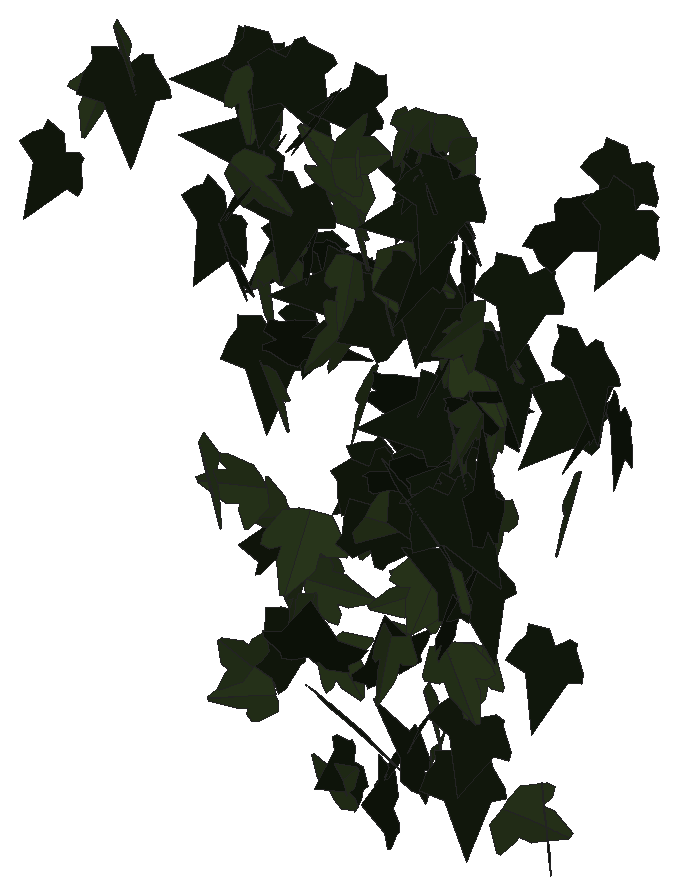
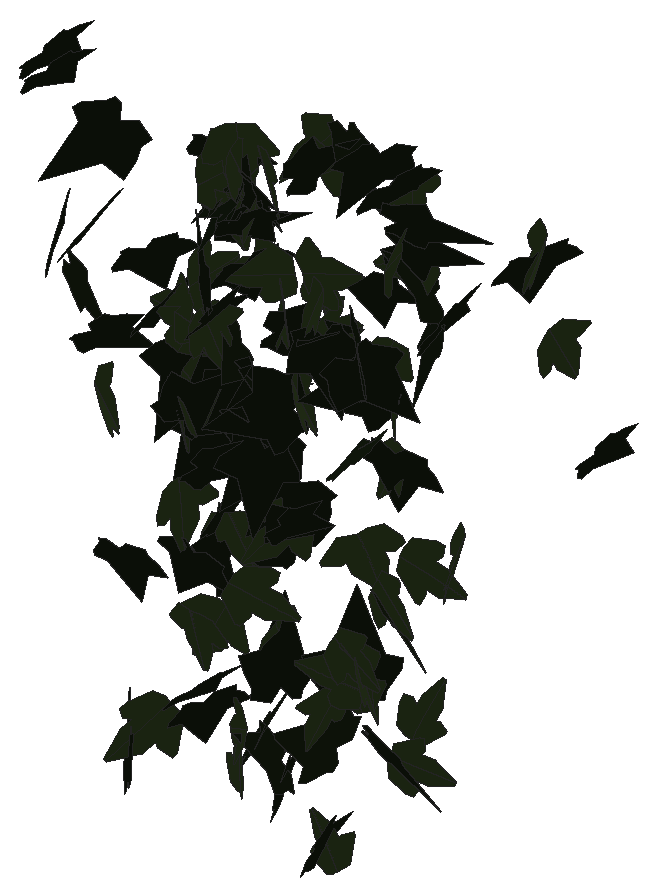
# SketchUp Ruby script. Lengths in inches.
U = 1.inch
M = Sketchup.active_model
def pt(a) = Geom::Point3d.new(a.map { |v| v * U })
def face(e, loops, mat)
  f = e.add_face(loops[0].map { |a| pt(a) })
  loops[1..].each { |l| e.add_face(l.map { |a| pt(a) }).erase! }
  f.material = f.back_material = mat if mat
  f
end
# faces: each face lists its corners as indices into pts; further lists are holes
def faces(e, pts, list, mat = nil) = list.each { |f| face(e, (f[0].is_a?(Array) ? f : [f]).map { |l| l.map { |i| pts[i] } }, mat) }
# xy, xz, yz: faces in a plane at the given z, y or x. An outline is a flat list of corners, or four numbers for a rectangle; further outlines are holes
def ring(l) = l.size == 4 ? [[l[0], l[1]], [l[2], l[1]], [l[2], l[3]], [l[0], l[3]]] : l.each_slice(2).to_a
def flat(e, list, mat, &to3) = list.each { |f| face(e, (f[0].is_a?(Array) ? f : [f]).map { |l| ring(l).map { |u, v| to3.(u, v) } }, mat) }
def xy(e, z, list, mat = nil) = flat(e, list, mat) { |x, y| [x, y, z] }
def xz(e, y, list, mat = nil) = flat(e, list, mat) { |x, z| [x, y, z] }
def yz(e, x, list, mat = nil) = flat(e, list, mat) { |y, z| [x, y, z] }
def lines(e, pts, list) = list.each { |a, b| e.add_line(pt(pts[a]), pt(pts[b])) }
# prism: a flat outline (further loops are holes) pulled along v
def prism(e, loops, v, mat = nil)
  f = face(e, loops, mat); d = Geom::Vector3d.new(v.map { |x| x * U })
  f.pushpull(f.normal.samedirection?(d) ? d.length : -d.length)
end
def box(e, o, s, mat = nil) = prism(e, [[o, [o[0] + s[0], o[1], o[2]], [o[0] + s[0], o[1] + s[1], o[2]], [o[0], o[1] + s[1], o[2]]]], [0, 0, s[2]], mat)
def at(x, y, z, deg = 0) = Geom::Transformation.translation(pt([x, y, z])) * Geom::Transformation.rotation(ORIGIN, Z_AXIS, deg.degrees)
def axes(o, x, y, z) = Geom::Transformation.new([*x, 0, *y, 0, *z, 0, *pt(o).to_a, 1])
def part(name) = M.definitions.add(name)
# library, detail: a bought-in or finely detailed component or shape, given as its bounding box
def library(name, o, s) = part(name).tap { |d| box(d.entities, o, s) }
def detail(e, o, s) = box(e.add_group.entities, o, s)
def put(e, d, t, mat = nil) = e.add_instance(d, t).tap { |i| i.material = mat if mat }
def group(e, t, mat = nil) = e.add_group.tap { |g| g.transformation = t; g.material = mat if mat }.entities
root = M.entities
M.materials.add("efeu1").color = [18, 25, 13]
M.materials.add("efeu2").color = [43, 57, 29]
c1 = part("ivyleaf_10")
p = [[0,0.5,-0.03],[-0.0625,2.02,-0.43],[-0.19,2.01,-0.46],[-0.54,1.05,-0.29],[-0.52,0.625,-0.18],[-0.83,0.76,-0.28],
  [-1.16,0.64,-0.33],[-1.15,0.33,-0.24],[-0.77,-0.39,0.02],[-0.3,-0.51,0.16],[0.04,-0.48,0.23],[-0.02,2.01,-0.4375],
  [-0.06,2.01,-0.43],[0.04,-0.49,0.23],[0.67,-0.49,0.14],[1.38,0.36,-0.2],[1.375,0.51,-0.24],[0.81,0.65,-0.19],
  [0.62,0.59,-0.15],[0.6,1.09,-0.28],[0.5,1.23,-0.31]]
faces(c1.entities,p,[[0,1,2,3,4,5,6,7,8,9,10],[11,12,0,13,14,15,16,17,18,19,20]],"efeu2")
c2 = part("ivyleaf_9")
p = [[1.54,2.16,1.25],[1.36,2.04,1.19],[-0.21,0.99,0.68],[-0.71,1.11,0.82],[-0.85,0.86,0.67],[-0.8,0.17,0.21],
  [-0.9,-0.01,0.1],[-0.67,-0.16,-0.02],[-0.08,-0.08,-0.05],[-0.03,-0.6,-0.4],[0.65,-0.88,-0.66],[0.83,-0.6,-0.49],
  [1.29,-0.42,-0.43],[1.8125,-0.07,-0.26],[1.21,0.44,0.15]]
faces(c2.entities,p,[[0,1,2,3,4,5,6,7,8,9,10,11,12,13,14]],"efeu1")
put(root,c1,axes([506.54,130.52,199.08],[-0.00627,-0.15637,0.93433],[0.25618,-0.86774,-0.15548],[0.95095,0.23273,0.04805]))
put(root,c1,axes([503.25,130.37,187.29],[-0.25922,-0.47722,-0.5607],[-0.25918,-0.48278,0.55554],[-0.73314,0.3394,0.00185]))
put(root,c1,axes([505.48,130.12,192.53],[0.69257,0.65461,-0.29515],[-0.19639,-0.21903,-0.95275],[-0.74512,0.66618,-0.02322]))
put(root,c2,axes([502.125,130.74,201.16],[-0.14431,-0.75939,0.55347],[-0.07524,-0.52794,-0.80165],[0.99866,-0.14951,0.01958]))
put(root,c1,axes([506.75,130.1,204.41],[0.54661,0.1085,0.66627],[-0.67489,-0.14122,0.5383],[0.19227,-0.80414,-0.00464]))
put(root,c2,axes([512.3,129.8,195.1],[-0.12147,-0.53915,0.79492],[0.15053,0.78066,0.55249],[-0.94864,0.19291,-0.01411]))
put(root,c1,axes([501.97,130.09,193.54],[-0.52665,0.83056,-0.10382],[0.04851,-0.08939,-1.00163],[-0.90216,-0.48966,0.00675]))
put(root,c2,axes([510.1,130.49,203.04],[-0.89494,0.25895,-0.37431],[0.36721,-0.1185,-0.90282],[-0.30734,-0.89562,0.01123]))
put(root,c1,axes([506.82,130.43,201.11],[0.79198,-0.33689,0.12485],[0.11865,-0.04842,-0.83928],[0.36757,0.7415,0.00191]))
put(root,c2,axes([505.98,130.14,205.92],[-0.44026,0.68291,-0.04296],[0.01968,-0.03722,-0.82713],[-0.73863,-0.40804,0.00356]))
put(root,c2,axes([508.62,130.63,194.77],[0.64339,-0.64937,0.36279],[0.24199,-0.27085,-0.91396],[0.70338,0.68717,-0.01741]))
put(root,c2,axes([516.2,130.92,199.53],[0.14807,-0.04382,-0.8756],[0.76524,-0.42684,0.15077],[-0.42778,-0.77872,-0.03337]))
put(root,c2,axes([505.23,130.65,188.13],[0.95979,0.11256,0.3282],[-0.33969,-0.02795,0.93156],[0.12468,-0.94265,0.01157]))
put(root,c1,axes([503.05,130.43,203.03],[-0.43402,0.06889,-0.75913],[0.77065,-0.15446,-0.42374],[-0.1819,-0.8188,0.01606]))
put(root,c2,axes([498.62,130.75,204.66],[-0.16588,-0.89543,-0.19328],[0.03476,0.18304,-0.94485],[0.98706,-0.15692,0.00079]))
put(root,c2,axes([502.73,130.12,200.56],[0.58447,-0.12641,-0.61836],[-0.60118,0.21677,-0.57485],[0.26375,0.77421,0.05999]))
put(root,c1,axes([507.24,129.79,205.2],[-0.0469,0.24958,0.915],[-0.14978,0.86881,-0.26344],[-0.97626,-0.14529,-0.00354]))
put(root,c1,axes([503.45,130.76,186.16],[-0.14934,-0.06886,0.76036],[-0.64128,-0.42726,-0.15865],[0.46665,-0.60918,0.02532]))
put(root,c2,axes([510.42,130.52,195],[-0.10303,-0.62569,-0.77186],[0.22837,0.74031,-0.6306],[0.96701,-0.2415,0.06668]))
put(root,c1,axes([503.16,130.58,192.85],[0.2711,0.0248,-0.88644],[-0.89864,0.2014,-0.24876],[0.20136,0.86542,0.08329]))
put(root,c2,axes([504.47,130.32,198.14],[0.69471,0.11427,0.57608],[0.58552,0.11438,-0.6793],[-0.174,0.84114,0.01411]))
put(root,c2,axes([507.66,131.34,183.74],[-0.1091,-0.08229,0.88592],[-0.16315,-0.84258,-0.10328],[0.90977,-0.16097,0.08772]))
put(root,c1,axes([507.06,131.08,197.43],[0.42021,-0.70124,0.3639],[0.17987,-0.30775,-0.83402],[0.82706,0.42321,-0.00351]))
put(root,c2,axes([502.77,130.29,201.88],[-0.26316,0.8029,-0.00051],[-0.00171,0.00003,0.87262],[0.86713,0.24367,0.00157]))
put(root,c1,axes([509.53,130.91,192.0625],[0.94419,0.18143,-0.25095],[-0.26115,-0.02177,-0.92817],[-0.1952,0.90668,0.02793]))
put(root,c2,axes([510.12,131.34,191.86],[0.09868,-0.82641,-0.19607],[0.14463,-0.17316,0.85693],[-0.90395,-0.11792,0.1157]))
put(root,c1,axes([510.5,131.54,200.18],[-0.02299,0.06424,-0.93277],[-0.20038,-0.91171,-0.05785],[-0.91326,0.19842,0.03617]))
put(root,c2,axes([503.25,131.15,203.67],[-0.32549,-0.30472,-0.72787],[-0.50672,-0.51958,0.44539],[-0.65028,0.55739,0.01726]))
put(root,c2,axes([509.9,131.2,204.73],[-0.75908,-0.48965,-0.2626],[0.23335,0.13151,-0.89073],[0.54732,-0.73516,0.01556]))
put(root,c1,axes([503,130.95,205.71],[0.38396,0.75556,-0.13563],[-0.05574,-0.11985,-0.86841],[-0.82619,0.35922,-0.00444]))
put(root,c2,axes([516.15,131.59,205.78],[-0.26948,-0.81812,0.36655],[-0.08715,-0.35704,-0.86095],[0.89224,-0.28197,0.02662]))
put(root,c1,axes([507.8,131.2,189.28],[0.00028,0.76902,-0.48897],[-0.0937,-0.46796,-0.79608],[-0.96895,0.04547,0.07685]))
put(root,c1,axes([498.27,130.91,205.31],[-0.57945,0.73808,-0.20405],[0.14171,-0.14713,-0.94878],[-0.81255,-0.55201,-0.01996]))
put(root,c2,axes([510.43,131.28,185.92],[-0.18672,-0.81634,-0.15457],[0.02994,0.14605,-0.86782],[0.89564,-0.17507,-0.00321]))
put(root,c2,axes([507.49,131.5,199.46],[-0.53265,-0.29506,0.65508],[-0.59107,-0.31194,-0.59763],[0.46362,-0.73667,-0.00932]))
put(root,c1,axes([503.56,130.97,196.34],[-0.62528,0.43595,-0.23173],[0.19667,-0.12856,-0.7537],[-0.49082,-0.60689,-0.00679]))
put(root,c2,axes([509.6,131.56,196.77],[-0.48618,-0.21057,0.75866],[-0.70519,-0.28011,-0.52965],[0.35018,-0.85644,-0.0133]))
put(root,c2,axes([510.26,130.43,190.5],[0.11335,0.00202,0.90987],[0.26812,0.84486,-0.033],[-0.90603,0.25027,0.10406]))
put(root,c2,axes([508.74,131.44,201.26],[-0.24656,-0.83402,-0.09447],[0.01607,0.0901,-0.89924],[0.90593,-0.22859,-0.00976]))
put(root,c2,axes([508.31,130.57,195.15],[0.6924,0.59926,0.18314],[0.13825,0.12093,-0.91268],[-0.66025,0.65376,0.00095]))
put(root,c2,axes([504.25,131.4375,202.31],[-0.68551,-0.47681,-0.36063],[0.3347,0.16361,-0.82394],[0.54167,-0.70453,0.05272]))
put(root,c2,axes([505.58,131.34,186.21],[0.57361,-0.60244,0.47494],[0.49041,-0.19197,-0.81262],[0.65275,0.67363,0.19317]))
put(root,c2,axes([503.875,130.96,191.2],[-0.49109,0.52248,0.28643],[-0.19842,0.20521,-0.72033],[-0.60623,-0.49041,0.00374]))
put(root,c2,axes([514.4,131.66,200.69],[0.21824,-0.93251,0.16658],[0.04308,-0.161,-0.95769],[0.94629,0.22239,0.00518]))
put(root,c1,axes([503.86,131.2,191.9],[-0.38111,0.07422,0.72466],[-0.75296,0.04119,-0.37176],[-0.07603,-0.77996,0.04932]))
put(root,c2,axes([508.51,131.59,185.2],[0.1339,-0.85102,0.27522],[-0.04293,0.27185,0.86149],[-0.89339,-0.14062,-0.00014]))
put(root,c1,axes([503.66,130.84,198.33],[-0.14548,0.3733,-0.80448],[-0.36571,0.69649,0.41089],[0.85248,0.3625,0.03898]))
put(root,c1,axes([509.76,131.48,189.2],[-0.87779,-0.11114,-0.3883],[0.42066,-0.24712,-0.80529],[-0.00744,-0.85961,0.28171]))
put(root,c2,axes([506.98,131.26,194.42],[-0.22448,-0.32486,-0.82506],[0.462,0.66812,-0.40109],[0.80234,-0.4756,0.00011]))
put(root,c2,axes([507.28,130.96,192.22],[-0.26623,-0.15936,0.89671],[0.80187,0.4385,0.30505],[-0.50374,0.78225,0.01168]))
put(root,c1,axes([507.79,131.09,201.11],[0.11805,0.09762,0.89752],[0.74462,0.51919,-0.1519],[-0.57041,0.69797,-0.01254]))
put(root,c2,axes([503.93,131.33,206.51],[-0.01865,-0.64039,-0.64725],[0.06645,0.62014,-0.66541],[0.96213,-0.05524,0.03341]))
put(root,c2,axes([507.25,131.71,187.92],[0.49185,0.45828,0.63564],[-0.44533,-0.45154,0.67164],[0.69453,-0.61407,-0.0195]))
put(root,c2,axes([502.94,131.95,206.09],[-0.23572,-0.86858,0.03156],[-0.01098,-0.02873,-0.9314],[0.93857,-0.21848,-0.00297]))
put(root,c1,axes([509.73,131.54,196.77],[-0.3781,0.73831,-0.28538],[0.15531,-0.23533,-0.84931],[-0.83637,-0.37747,-0.0287]))
put(root,c2,axes([509.5,130.82,198.05],[0.02693,0.50113,0.7574],[-0.03256,0.72861,-0.52036],[-0.9542,-0.01072,0.03914]))
put(root,c1,axes([504.3,131.64,188.41],[-0.71935,0.12347,0.36223],[0.36944,-0.06554,0.70451],[0.15095,0.74877,0.00194]))
put(root,c1,axes([507.36,131.04,193.1],[-0.28697,-0.47046,-0.793],[0.46421,0.64387,-0.54998],[0.79668,-0.54464,0.03482]))
put(root,c1,axes([510.29,132.01,197.08],[0.04885,-0.70836,0.54054],[0.07793,-0.51569,-0.73747],[0.94567,0.07909,0.03285]))
put(root,c1,axes([496.8,131.97,203.13],[-0.18194,-0.69428,0.42901],[0.11926,-0.45744,-0.68972],[0.80738,-0.08888,0.19855]))
put(root,c1,axes([507.73,131.11,200.02],[-0.06734,0.04516,0.91041],[-0.78206,0.49188,-0.08003],[-0.53346,-0.72681,0.0024]))
put(root,c2,axes([502.93,131.79,197.03],[-0.67415,-0.37545,-0.54501],[0.48426,0.27124,-0.75756],[0.50022,-0.76857,-0.00111]))
put(root,c1,axes([503.57,131.32,200.03],[-0.35478,-0.52431,-0.45713],[0.27599,0.35827,-0.64308],[0.68544,-0.41564,0.02233]))
put(root,c2,axes([495.1,132.2,200.04],[-0.22493,-0.6929,0.37191],[-0.13078,-0.34848,-0.72834],[0.77545,-0.25976,-0.01496]))
put(root,c2,axes([508.75,132.16,202.8],[-0.52454,-0.17652,0.66201],[-0.54027,-0.41769,-0.51742],[0.4659,-0.68309,0.14532]))
put(root,c2,axes([509.41,131.3,195.33],[-0.91543,0.11244,-0.06237],[-0.06418,-0.01097,0.92212],[0.11142,0.91749,0.01867]))
put(root,c2,axes([506.22,132.25,205.43],[-0.17052,-0.20215,0.74868],[-0.53535,-0.52255,-0.26567],[0.60459,-0.51971,-0.02409]))
put(root,c2,axes([505.78,132.08,199.39],[-0.51164,-0.13803,0.6595],[-0.65599,-0.1822,-0.51317],[0.24684,-0.7703,0.0032]))
put(root,c2,axes([511.34,132.09,199.34],[0.13291,-0.88117,0.07294],[0.00441,-0.07024,-0.92529],[0.95466,0.123,-0.00588]))
put(root,c2,axes([510.03,132.28,186.97],[-0.26754,-0.79881,0.25127],[0.09087,-0.27464,-0.85466],[0.89672,-0.21049,0.16157]))
put(root,c2,axes([514.9,131.82,199.06],[-0.66036,0.45424,-0.35024],[0.29848,-0.18394,-0.80134],[-0.48981,-0.7245,-0.01614]))
put(root,c2,axes([512.97,131.97,190.42],[-0.68012,-0.34453,-0.35706],[0.3136,0.17101,-0.76234],[0.38451,-0.74887,-0.00982]))
put(root,c1,axes([508.46,131.93,190.73],[0.38699,0.17423,-0.77875],[-0.80008,-0.14261,-0.40319],[-0.22197,0.81777,0.0956]))
put(root,c2,axes([507.66,131.27,185],[-0.32894,0.71407,-0.13413],[-0.05635,0.11796,0.80736],[0.78164,0.30901,0.00176]))
put(root,c2,axes([508.97,131.85,204.21],[0.57918,-0.66525,-0.12506],[-0.08983,0.08739,-0.88861],[0.72457,0.5426,-0.0102]))
put(root,c2,axes([507.18,131.43,196.94],[0.75847,0.0892,0.50625],[0.51946,0.07585,-0.73614],[-0.12578,0.85112,0.01255]))
put(root,c2,axes([502.5,132.08,205.08],[-0.69117,0.04553,0.64524],[-0.67167,-0.06786,-0.66199],[0.01588,-0.88875,0.0836]))
put(root,c2,axes([509.48,132.5,199.54],[-0.30863,-0.49948,0.63626],[-0.19378,-0.59254,-0.59027],[0.83067,-0.3238,0.0987]))
put(root,c2,axes([503.6,131.88,187.33],[-0.9004,0.31047,0.13101],[-0.12195,0.05769,-0.9251],[-0.34069,-0.84119,-0.01509]))
put(root,c1,axes([513.44,132.26,195.66],[0.48957,-0.67898,0.4519],[0.26538,-0.36577,-0.83707],[0.77123,0.55687,0.00117]))
put(root,c1,axes([503.93,132.07,189.75],[0.37659,-0.80897,0.13353],[0.05548,-0.11767,-0.91616],[0.88288,0.35246,0.00061]))
put(root,c1,axes([505.52,131.54,187.82],[0.15408,0.68944,0.36686],[0.03961,0.35227,-0.73146],[-0.83546,0.14385,0.03298]))
put(root,c1,axes([510.19,132,189.06],[0.89073,-0.10157,0.02006],[0.02086,-0.00097,-0.86422],[0.10969,0.82498,0.00146]))
put(root,c1,axes([512.03,131.45,185.07],[-0.34522,-0.48241,-0.78392],[0.53944,0.57236,-0.58977],[0.74582,-0.63727,0.06372]))
put(root,c1,axes([509.61,132.19,199.34],[-0.16771,-0.74784,0.28863],[0.01001,-0.28441,-0.79165],[0.86143,-0.14229,0.06539]))
put(root,c1,axes([510.28,131.875,198.77],[0.77579,0.2612,0.49274],[0.48692,0.14631,-0.79478],[-0.32298,0.84797,-0.01465]))
put(root,c2,axes([508.31,132.18,204.64],[-0.79801,0.02064,-0.29269],[0.30225,-0.04743,-0.76779],[-0.03903,-0.78926,0.03849]))
put(root,c2,axes([506.55,132.48,193.77],[-0.38252,-0.48743,0.40205],[-0.25705,-0.30484,-0.62652],[0.62078,-0.42658,-0.01169]))
put(root,c1,axes([510.47,132.17,199.21],[0.03764,-0.1215,0.84681],[0.87988,-0.1121,-0.05366],[0.12785,0.80724,0.12]))
put(root,c2,axes([508.28,132.3125,203.95],[0.02525,-0.00158,0.83928],[0.42708,-0.70375,-0.01335],[0.75976,0.39565,-0.02039]))
put(root,c1,axes([507.6875,131.92,205.31],[0.52664,-0.54317,-0.32544],[-0.20742,0.24794,-0.75883],[0.64445,0.52367,0.02171]))
put(root,c1,axes([502.48,132.56,203.78],[-0.07664,-0.23699,0.81822],[0.54404,-0.64577,-0.13608],[0.65548,0.50827,0.20861]))
put(root,c2,axes([508.37,132.56,204.29],[0.03675,-0.78678,0.33332],[0.09858,-0.31551,-0.8156],[0.91221,0.06579,0.07471]))
put(root,c1,axes([509.18,132.69,204.53],[-0.06704,0.01468,-0.90738],[-0.34999,-0.83989,0.01228],[-0.8373,0.34989,0.06753]))
put(root,c1,axes([505.76,132.07,202.21],[0.33252,0.07041,0.85628],[-0.83197,-0.20282,0.33976],[0.21448,-0.89591,-0.00962]))
put(root,c2,axes([504.55,131.6,200.57],[-0.16373,0.05141,-0.86151],[-0.84348,0.27615,0.16647],[0.30336,0.79557,-0.00211]))
put(root,c1,axes([504.92,132.14,183.08],[-0.60611,-0.01608,0.49767],[0.51682,0.00559,0.58387],[-0.01713,0.73751,0.00642]))
put(root,c2,axes([510.34,131.66,197.58],[0.77444,0.53301,-0.07329],[-0.05268,-0.0525,-0.92912],[-0.57827,0.71862,-0.01352]))
put(root,c1,axes([508.29,132.46,205.28],[0.17083,-0.7471,0.35],[0.127,-0.32935,-0.76501],[0.81518,0.20788,0.04584]))
put(root,c1,axes([507.97,132.3125,203.89],[-0.3899,0.42812,-0.53055],[0.37551,-0.37375,-0.58211],[-0.61346,-0.50088,-0.01912]))
put(root,c1,axes([508.57,132.15,205.78],[-0.7896,-0.41645,0.13607],[-0.12337,-0.06381,-0.87506],[0.45501,-0.73998,-0.00112]))
put(root,c2,axes([509.96,132.37,191.55],[-0.44584,-0.33258,-0.6574],[0.62684,0.26932,-0.54158],[0.4496,-0.7053,0.10319]))
put(root,c2,axes([513.35,132.76,197.98],[-0.57263,-0.55615,0.3063],[-0.21312,-0.22018,-0.79821],[0.59809,-0.61094,0.00884]))
put(root,c1,axes([508.13,132.62,184.77],[0.15096,-0.45966,-0.57067],[0.1748,-0.52431,0.49966],[-0.75305,-0.21385,0.00158]))
put(root,c2,axes([505.07,132.79,183.62],[0.23161,-0.4111,-0.57477],[0.35736,-0.44618,0.4787],[-0.65244,-0.39032,0.05816]))
put(root,c2,axes([509.36,132.8,194.85],[-0.50118,-0.45279,0.51307],[-0.38825,-0.33794,-0.67425],[0.61014,-0.58697,-0.0076]))
put(root,c1,axes([508.56,132.34,203.76],[0.85151,0.1008,-0.08604],[-0.08988,-0.00138,-0.82659],[-0.10843,0.79276,0.0095]))
put(root,c2,axes([508.31,132.41,204.27],[0.56294,-0.58551,0.07353],[0.05348,-0.05058,-0.81526],[0.6347,0.52357,0.00347]))
put(root,c2,axes([503.69,132.59,200.22],[0.06022,0.27157,-0.84205],[-0.23153,-0.78096,-0.28778],[-0.89279,0.22085,0.01783]))
put(root,c2,axes([509.34,132.6,200.44],[-0.16723,0.29273,0.80374],[0.13869,-0.7682,0.32938],[0.88168,0.17637,0.10064]))
put(root,c2,axes([512.11,132.77,183.67],[-0.09343,0.11907,0.88174],[0.10189,-0.87932,0.12954],[0.88389,0.11395,0.07827]))
put(root,c2,axes([507.62,132.05,195.64],[0.64101,0.44665,-0.41392],[-0.35977,-0.21894,-0.77218],[-0.53667,0.68025,0.02325]))
put(root,c2,axes([510.01,132.68,196.26],[0.15161,0.04258,0.85381],[-0.86654,-0.17427,0.15209],[0.19334,-0.81446,0.01209]))
put(root,c1,axes([504.45,132.38,190.31],[-0.39194,-0.06587,0.68595],[-0.69599,-0.14093,-0.3834],[0.16755,-0.7395,0.01196]))
put(root,c1,axes([505.45,132.35,201.68],[-0.59256,0.52702,-0.19064],[0.13347,-0.13593,-0.79111],[-0.58767,-0.56228,0.01256]))
put(root,c2,axes([513.34,131.75,204.45],[-0.01849,0.04954,-0.95837],[0.01449,0.95845,0.04927],[0.95954,-0.01352,-0.01921]))
put(root,c2,axes([507.82,132.87,203.65],[-0.4949,-0.62219,0.07269],[0.02549,-0.10372,-0.79929],[0.67571,-0.45179,0.08339]))
put(root,c1,axes([510.41,132.58,196.62],[0.74439,-0.51333,0.12873],[0.11608,-0.06288,-0.89367],[0.55835,0.69745,0.01417]))
put(root,c2,axes([514.92,132.96,206.21],[-0.26216,-0.79199,0.19051],[-0.00662,-0.19805,-0.83246],[0.81455,-0.2565,0.05455]))
put(root,c2,axes([508.52,132.25,204.28],[0.69397,-0.33376,-0.36161],[-0.33951,0.149,-0.75294],[0.39455,0.71525,-0.01189]))
put(root,c1,axes([507.93,132.71,186.62],[-0.22199,0.31364,-0.65053],[0.38819,-0.51203,-0.38985],[-0.64839,-0.41393,-0.01068]))
put(root,c1,axes([510.31,132.54,193.53],[-0.24714,-0.83236,0.0504],[0.13639,-0.08428,-0.88522],[0.89009,-0.2182,0.14964]))
put(root,c2,axes([511.34,132.83,201.42],[-0.3863,-0.80004,-0.10881],[0.03552,0.10366,-0.88833],[0.80662,-0.38771,-0.01299]))
put(root,c2,axes([503.59,133.05,197.11],[-0.13379,-0.65206,0.43289],[0.16255,-0.45274,-0.63173],[0.76561,-0.01782,0.20977]))
put(root,c2,axes([505.22,132.27,200.31],[0.33202,0.46958,-0.55991],[-0.53197,-0.28518,-0.55121],[-0.55882,0.55048,0.19206]))
put(root,c1,axes([504.15,132.38,189.25],[-0.10417,-0.02124,0.90496],[0.90049,0.24904,0.10244],[-0.26983,0.83931,-0.0075]))
